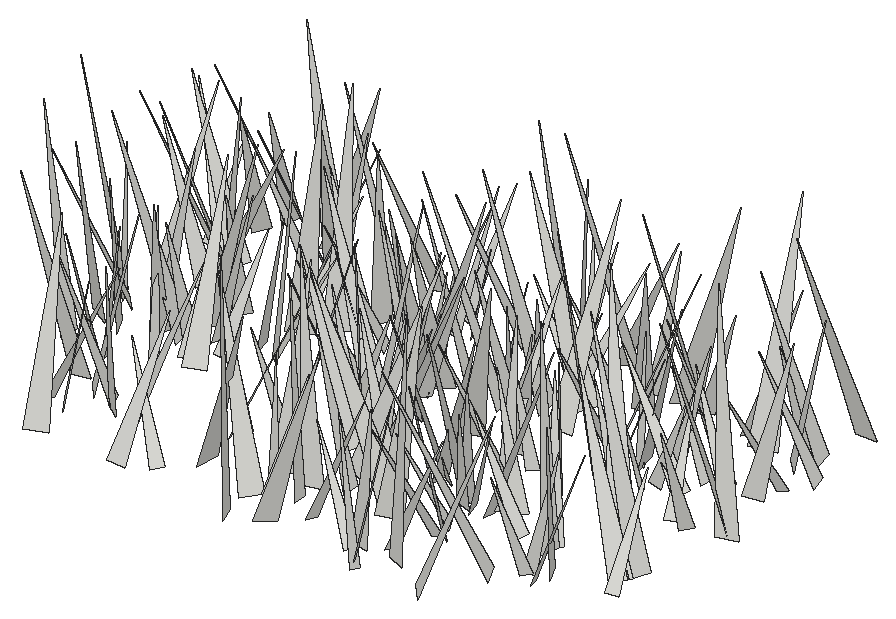
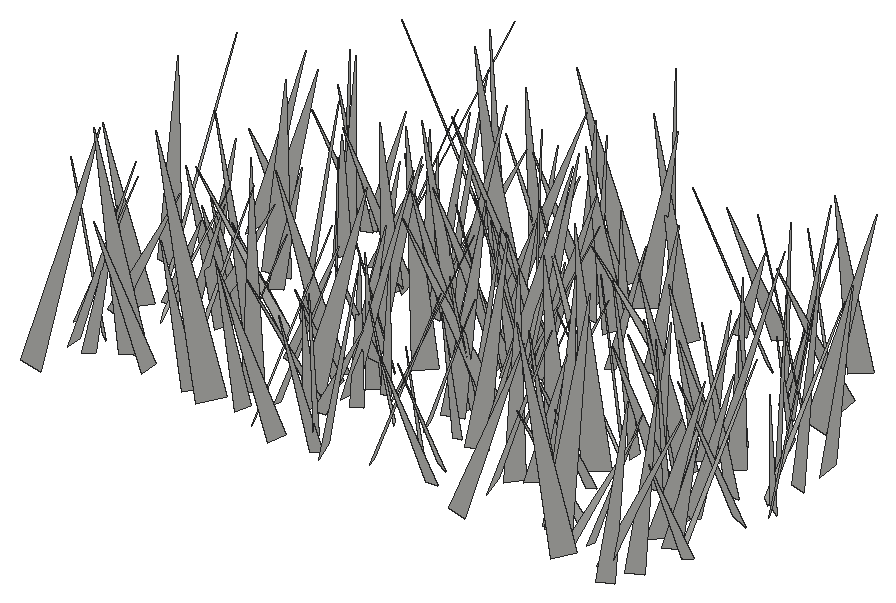
# SketchUp Ruby script. Lengths in inches.
U = 1.inch
M = Sketchup.active_model
def pt(a) = Geom::Point3d.new(a.map { |v| v * U })
def face(e, loops, mat)
  f = e.add_face(loops[0].map { |a| pt(a) })
  loops[1..].each { |l| e.add_face(l.map { |a| pt(a) }).erase! }
  f.material = f.back_material = mat if mat
  f
end
# faces: each face lists its corners as indices into pts; further lists are holes
def faces(e, pts, list, mat = nil) = list.each { |f| face(e, (f[0].is_a?(Array) ? f : [f]).map { |l| l.map { |i| pts[i] } }, mat) }
# xy, xz, yz: faces in a plane at the given z, y or x. An outline is a flat list of corners, or four numbers for a rectangle; further outlines are holes
def ring(l) = l.size == 4 ? [[l[0], l[1]], [l[2], l[1]], [l[2], l[3]], [l[0], l[3]]] : l.each_slice(2).to_a
def flat(e, list, mat, &to3) = list.each { |f| face(e, (f[0].is_a?(Array) ? f : [f]).map { |l| ring(l).map { |u, v| to3.(u, v) } }, mat) }
def xy(e, z, list, mat = nil) = flat(e, list, mat) { |x, y| [x, y, z] }
def xz(e, y, list, mat = nil) = flat(e, list, mat) { |x, z| [x, y, z] }
def yz(e, x, list, mat = nil) = flat(e, list, mat) { |y, z| [x, y, z] }
def lines(e, pts, list) = list.each { |a, b| e.add_line(pt(pts[a]), pt(pts[b])) }
# prism: a flat outline (further loops are holes) pulled along v
def prism(e, loops, v, mat = nil)
  f = face(e, loops, mat); d = Geom::Vector3d.new(v.map { |x| x * U })
  f.pushpull(f.normal.samedirection?(d) ? d.length : -d.length)
end
def box(e, o, s, mat = nil) = prism(e, [[o, [o[0] + s[0], o[1], o[2]], [o[0] + s[0], o[1] + s[1], o[2]], [o[0], o[1] + s[1], o[2]]]], [0, 0, s[2]], mat)
def at(x, y, z, deg = 0) = Geom::Transformation.translation(pt([x, y, z])) * Geom::Transformation.rotation(ORIGIN, Z_AXIS, deg.degrees)
def axes(o, x, y, z) = Geom::Transformation.new([*x, 0, *y, 0, *z, 0, *pt(o).to_a, 1])
def part(name) = M.definitions.add(name)
# library, detail: a bought-in or finely detailed component or shape, given as its bounding box
def library(name, o, s) = part(name).tap { |d| box(d.entities, o, s) }
def detail(e, o, s) = box(e.add_group.entities, o, s)
def put(e, d, t, mat = nil) = e.add_instance(d, t).tap { |i| i.material = mat if mat }
def group(e, t, mat = nil) = e.add_group.tap { |g| g.transformation = t; g.material = mat if mat }.entities
root = M.entities
c1 = part("fur_instance\#9")
p = [[0.8125,0,1.79],[0.67,-0.02,1.48],[0,-0.11,0],[0,0.11,0]]
faces(c1.entities,p,[[0,1,2,3]])
put(root,c1,axes([477.54,253.75,-21.66],[5.60342,-3.67276,1.04707],[-3.81273,-5.48708,1.15708],[-0.22057,1.54484,6.59914]))
put(root,c1,axes([489.59,252.63,-21.66],[4.90909,4.36789,0.50992],[4.39704,-4.86378,-0.66882],[0.06695,-0.83837,6.53684]))
put(root,c1,axes([475.34,252.89,-21.66],[-6.98093,-2.98191,2.95578],[-3.56155,7.24267,-1.10492],[2.22346,2.23913,7.51028]))
put(root,c1,axes([485.04,252.59,-21.66],[-4.58169,-0.00231,0.33908],[-0.10273,4.38765,-1.35823],[0.32316,1.36211,4.37574]))
put(root,c1,axes([483.6,254.77,-21.66],[0.23103,-4.99246,1.62863],[-5.17408,0.0623,0.92493],[0.89778,1.64376,4.91147]))
put(root,c1,axes([483.45,254.25,-21.66],[-2.38468,3.13652,0.12042],[3.02513,2.25628,1.13874],[-0.83714,-0.7813,3.77197]))
put(root,c1,axes([491.6,256.91,-21.66],[-6.74137,-3.47517,0.05647],[-3.44773,6.70195,0.85032],[0.43951,-0.73012,7.53656]))
put(root,c1,axes([484.39,253.45,-21.66],[3.67967,2.76321,1.03507],[2.46473,-3.78797,1.35021],[-1.62229,0.51247,4.39911]))
put(root,c1,axes([466.65,253.6,-21.66],[-1.32926,4.80497,0.97182],[4.66035,1.55098,-1.29408],[1.52094,-0.553,4.81456]))
put(root,c1,axes([460.62,253.74,-21.66],[-3.43213,5.64571,1.59286],[5.69776,3.64732,-0.65059],[1.39526,-1.00684,6.57497]))
put(root,c1,axes([468.8125,254.67,-21.66],[-2.26305,3.25436,0.20739],[3.19812,2.16563,0.91504],[-0.63708,-0.68879,3.8568]))
put(root,c1,axes([486.45,254.625,-21.66],[3.17531,6.56755,2.54139],[6.79761,-3.58673,0.77578],[-1.83954,-1.91744,7.25351]))
put(root,c1,axes([470.55,257.12,-21.66],[6.6655,-1.52718,0.22941],[-1.49066,-6.62814,-0.81212],[-0.40351,-0.74118,6.78982]))
put(root,c1,axes([485.29,255.67,-21.66],[4.11337,-1.35782,0.42666],[-1.42017,-4.00175,0.95638],[-0.09392,1.04301,4.22479]))
put(root,c1,axes([475.1,255.56,-21.66],[-5.2406,4.407,1.34408],[4.57378,5.22157,0.71269],[0.55566,-1.41624,6.81011]))
put(root,c1,axes([479.43,255.63,-21.66],[4.44559,-0.41699,0.42413],[-0.48383,-4.39553,0.74982],[-0.34594,0.78895,4.4017]))
put(root,c1,axes([459.94,257.18,-21.66],[4.41125,2.39111,1.26664],[2.67652,-4.21168,-1.37073],[-0.39751,-1.82353,4.82677]))
put(root,c1,axes([475.95,255.86,-21.66],[1.17442,4.10835,0.87727],[4.16659,-1.02282,-0.78793],[0.5364,-1.0501,4.19964]))
put(root,c1,axes([493.22,258.1875,-21.66],[1.75124,-3.26229,0.83742],[-3.12175,-1.92651,-0.97669],[-1.26432,0.23809,3.57148]))
put(root,c1,axes([486.37,258.55,-21.66],[-0.29394,-4.28793,0.2812],[-4.0742,0.18848,-1.38464],[-1.36614,0.36048,4.06885]))
put(root,c1,axes([486.57,258.94,-21.66],[-3.34858,-4.98605,1.16696],[-4.83329,3.53804,1.24784],[1.69169,0.23891,5.87509]))
put(root,c1,axes([462.59,258.34,-21.66],[-2.53313,-4.37285,1.78451],[-4.47538,2.86942,0.67851],[1.50904,1.16947,5.00781]))
put(root,c1,axes([475.53,256.97,-21.66],[-3.90689,0.46662,1.17538],[0.26281,4.03296,-0.72751],[1.23701,0.61693,3.86682]))
put(root,c1,axes([465.07,256.54,-21.66],[3.93505,4.96293,0.50565],[4.97977,-3.8695,-0.7745],[0.29702,-0.87596,6.28613]))
put(root,c1,axes([462.05,259.17,-21.66],[-5.06877,-1.96642,0.89661],[-1.81084,5.11214,0.97466],[1.17965,-0.60192,5.34876]))
put(root,c1,axes([477.48,256.97,-21.66],[-6.31895,-1.30533,1.91515],[-1.71826,6.37081,-1.32708],[1.5554,1.73484,6.31441]))
put(root,c1,axes([460.6,260.3,-21.66],[-3.28751,-5.48957,1.02333],[-5.33666,3.43821,1.29963],[1.64396,0.18343,6.2653]))
put(root,c1,axes([494.35,259.13,-21.66],[-4.3896,-2.50757,2.34029],[-2.3133,4.97071,0.98703],[2.5325,0.19407,4.95805]))
put(root,c1,axes([458.72,257.25,-21.66],[4.92318,-0.35306,0.35659],[-0.43613,-4.74982,1.31852],[-0.24819,1.34315,4.75646]))
put(root,c1,axes([493.17,258.53,-21.66],[0.04539,-4.24616,1.86431],[-4.44886,0.48634,1.21602],[1.30888,1.80033,4.06857]))
put(root,c1,axes([482.85,258.52,-21.66],[-2.73382,6.12597,3.74599],[6.6709,3.64992,-1.10045],[2.6569,-2.86083,6.61742]))
put(root,c1,axes([486.19,259.98,-21.66],[-3.41179,-1.77285,0.16017],[-1.67154,3.30984,1.02951],[0.61205,-0.84317,3.70451]))
put(root,c1,axes([479.12,259.64,-21.66],[-5.12264,0.34016,1.65759],[0.60899,5.30124,0.79415],[1.57874,-0.94118,5.07212]))
put(root,c1,axes([494.16,257.65,-21.66],[3.89284,1.77366,0.49192],[1.64576,-3.86945,0.92782],[-0.82421,0.65077,4.17603]))
put(root,c1,axes([458.6,260.4,-21.66],[-0.74223,-7.02206,1.66779],[-7.14663,0.48084,-1.156],[-1.00829,1.76103,6.96591]))
put(root,c1,axes([477.17,258.53,-21.66],[-0.74799,6.94474,2.29097],[7.27165,0.46217,0.97314],[-0.77532,-2.36525,6.91678]))
put(root,c1,axes([481.41,260.32,-21.66],[-7.37091,1.53228,0.84327],[1.65266,7.29739,1.18581],[0.57246,-1.33774,7.43452]))
put(root,c1,axes([460.25,259.54,-21.66],[4.87544,3.99495,1.42226],[4.19795,-4.85335,-0.75795],[-0.59966,-1.4959,6.2574]))
put(root,c1,axes([474.77,258.71,-21.66],[-5.03968,3.97301,2.20808],[3.85689,5.48236,-1.06156],[2.40517,-0.46656,6.329]))
put(root,c1,axes([485.34,262.1875,-21.66],[-0.07367,-4.26522,0.50041],[-4.16979,0.19077,1.01214],[1.02732,0.46845,4.14405]))
put(root,c1,axes([469.96,261.27,-21.66],[-0.83956,4.61048,2.28414],[5.1209,0.52371,0.82514],[-0.50027,-2.37653,4.61309]))
put(root,c1,axes([498.55,259.42,-21.66],[-1.96871,3.37657,0.07437],[3.27614,1.93014,-0.90775],[0.82077,0.39482,3.80171]))
put(root,c1,axes([490.25,261.45,-21.66],[-3.73947,1.85603,0.44676],[1.90802,3.6015,1.00834],[-0.06253,-1.10111,4.05114]))
put(root,c1,axes([485.99,262.29,-21.66],[4.14097,0.37336,0.37849],[0.46882,-3.96604,-1.21698],[-0.25072,-1.24957,3.97567]))
put(root,c1,axes([472.2,262.34,-21.66],[-3.76395,0.54517,1.33918],[0.93594,3.7652,1.09781],[1.1021,-1.33566,3.64133]))
put(root,c1,axes([485.17,262.84,-21.66],[0.2797,-5.08952,0.70223],[-5.01624,-0.11848,1.13926],[1.11073,0.74654,4.96825]))
put(root,c1,axes([497.95,260.98,-21.66],[-4.76226,4.46867,0.77555],[4.53262,4.64929,1.04363],[-0.16086,-1.29026,6.44663]))
put(root,c1,axes([492.59,261.12,-21.66],[-6.8831,0.44539,2.18741],[0.27023,7.20464,-0.61666],[2.21588,0.50489,6.86987]))
put(root,c1,axes([482.55,264.125,-21.66],[-2.90954,-6.16313,0.64564],[-6.10361,2.97343,0.8781],[1.07095,0.20243,6.75859]))
put(root,c1,axes([469.79,260.22,-21.66],[4.40688,2.08061,0.00975],[2.02682,-4.29803,1.08102],[-0.47012,0.97349,4.75194]))
put(root,c1,axes([488.1,264.1,-21.66],[-5.70608,-2.81682,0.48614],[-2.67601,5.6456,1.30244],[1.0049,-0.96065,6.22877]))
put(root,c1,axes([483.9,264.02,-21.66],[-1.823,-5.96341,0.88128],[-5.94354,1.93183,0.77754],[1.00658,0.60664,6.18716]))
put(root,c1,axes([482.34,263.86,-21.66],[6.03259,-1.06555,0.38284],[-1.02373,-6.01977,-0.62323],[-0.48366,-0.54868,6.09418]))
put(root,c1,axes([492.49,261.68,-21.66],[-4.5808,2.50643,0.71678],[2.42315,4.62824,-0.69815],[0.96142,0.27723,5.1748]))
put(root,c1,axes([478.18,261.3,-21.66],[3.15625,6.97995,0.87784],[7.00121,-3.02246,-1.14023],[0.68808,-1.26383,7.57506]))
put(root,c1,axes([498.39,262.12,-21.66],[-7.87651,1.28049,0.44694],[1.23259,7.85729,-0.78901],[0.56579,0.70864,7.94081]))
put(root,c1,axes([476.51,263.96,-21.66],[-4.90081,-4.60842,2.76686],[-4.75517,5.4628,0.67611],[2.50627,1.35324,6.69315]))
put(root,c1,axes([488.52,263.48,-21.66],[-2.55012,3.64542,1.48438],[3.93085,2.44958,0.73729],[0.20222,-1.64502,4.38733]))
put(root,c1,axes([487.19,262.31,-21.66],[5.64038,0.84844,0.8162],[0.68974,-5.61874,1.07421],[-0.95409,0.95384,5.60177]))
put(root,c1,axes([478.86,263.42,-21.66],[-2.03282,4.17049,1.29504],[4.34211,1.77825,1.08919],[-0.46493,-1.62705,4.50988]))
put(root,c1,axes([476.25,263.72,-21.66],[-6.01632,2.22797,0.81671],[2.32649,5.97644,0.83455],[0.46722,-1.07014,6.36109]))
put(root,c1,axes([458.35,262.9,-21.66],[-3.5127,-1.06556,1.8883],[-1.54789,3.74984,-0.76344],[1.51826,1.35772,3.59049]))
put(root,c1,axes([487.5,263.29,-21.66],[4.97353,-2.18793,2.98402],[-2.79783,-5.49524,0.634],[-2.42149,1.85546,5.39639]))
put(root,c1,axes([454.93,263.9375,-21.66],[-7.05246,-0.20222,1.59365],[-0.38202,7.18084,-0.77939],[1.56034,0.84409,7.01218]))
put(root,c1,axes([454.98,266.61,-21.66],[-2.48382,-6.27006,1.58629],[-6.2632,2.75568,1.08533],[1.61318,1.04494,6.65621]))
put(root,c1,axes([476.97,265.03,-21.66],[3.46953,-2.67132,1.40146],[-2.94376,-3.4648,0.68347],[-0.65905,1.41311,4.3251]))
put(root,c1,axes([474.43,265.07,-21.66],[3.70527,-2.55389,0.75103],[-2.66189,-3.54115,1.0909],[0.02774,1.32414,4.36593]))
put(root,c1,axes([456.74,266.31,-21.66],[4.97052,1.68586,2.30908],[2.28367,-5.12743,-1.17229],[-1.72012,-1.9358,5.11604]))
put(root,c1,axes([460.83,264.32,-21.66],[0.97276,4.45119,0.9772],[4.35496,-1.20232,1.14148],[-1.3425,-0.67498,4.41093]))
put(root,c1,axes([459.04,267.11,-21.66],[4.90376,-2.85552,0.72078],[-2.73926,-4.93651,-0.92072],[-1.08166,-0.44414,5.59939]))
put(root,c1,axes([475.1,267.5,-21.66],[-5.50457,-1.9976,0.13924],[-1.94432,5.42927,1.02602],[0.47897,-0.91798,5.76524]))
put(root,c1,axes([474.72,265.8,-21.66],[0.57769,-3.84784,2.16026],[-4.16363,-1.197,-1.01866],[-1.46176,1.88882,3.75525]))
put(root,c1,axes([461.22,267.4375,-21.66],[3.60801,-2.69307,1.35493],[-2.4926,-3.85347,-1.02171],[-1.69571,-0.06573,4.3848]))
put(root,c1,axes([470.25,266.47,-21.66],[6.04949,2.12455,0.78775],[2.22415,-5.99674,-0.90711],[-0.43293,-1.1207,6.34722]))
put(root,c1,axes([455.41,268.98,-21.66],[-4.43936,-4.76816,0.23664],[-4.66276,4.39992,1.18262],[1.02469,-0.63608,6.40661]))
put(root,c1,axes([488.52,267.26,-21.66],[3.47548,2.68418,2.07766],[3.24177,-3.50628,-0.89294],[-1.00618,-2.02524,4.29959]))
put(root,c1,axes([460.34,267.6,-21.66],[-7.46338,-1.41905,1.28497],[-1.31215,7.55774,0.72509],[1.39396,-0.48353,7.56241]))
put(root,c1,axes([475.88,266.6,-21.66],[-6.89397,4.20656,1.53795],[4.42912,6.82252,1.19307],[0.66584,-1.82904,7.9874]))
put(root,c1,axes([477.26,265.78,-21.66],[6.02676,-0.13267,0.65935],[-0.25057,-5.95995,1.09109],[-0.62414,1.1116,5.92866]))
put(root,c1,axes([474.29,268.35,-21.66],[-3.67064,-4.64361,1.03864],[-4.58105,3.8034,0.81465],[1.28682,0.29416,5.86285]))
put(root,c1,axes([497.07,268.18,-21.66],[2.57242,-3.23839,0.522],[-3.12857,-2.6216,-0.84629],[-0.98573,-0.13048,4.04824]))
put(root,c1,axes([493.08,267.05,-21.66],[-3.28307,2.60382,1.30489],[2.8552,3.26547,0.66758],[0.57484,-1.34832,4.13676]))
put(root,c1,axes([462.01,265.79,-21.66],[-2.71251,3.20119,0.88639],[3.03008,2.85354,-1.03292],[1.36084,0.02704,4.06674]))
put(root,c1,axes([494.09,265.75,-21.66],[-3.06885,7.2619,1.47031],[7.40414,2.94663,0.90053],[-0.27521,-1.70206,7.83212]))
put(root,c1,axes([480.46,269.07,-21.66],[3.94338,-5.9757,0.15667],[-5.94055,-3.89659,0.90015],[0.66588,0.62564,7.10275]))
put(root,c1,axes([463.16,265.17,-21.66],[-3.56616,5.34471,0.77163],[5.27091,3.64619,-0.89538],[1.17426,-0.13507,6.36253]))
put(root,c1,axes([472.08,268.04,-21.66],[-2.77092,-3.22119,0.17285],[-3.17409,2.68192,-0.90354],[-0.57541,0.71776,4.15182]))
put(root,c1,axes([476.3,265.0625,-21.66],[3.93079,5.90323,1.06815],[5.73682,-4.07234,1.39466],[-1.7544,-0.09002,6.95371]))
put(root,c1,axes([477.33,266,-21.66],[-3.93965,-2.75758,3.63418],[-3.8658,4.56754,-0.72493],[2.42222,2.80458,4.7539]))
put(root,c1,axes([498.85,269.73,-21.66],[-5.87389,-5.06073,1.31002],[-4.91563,6.01764,1.20596],[1.77871,-0.08191,7.65893]))
put(root,c1,axes([485.84,268.02,-21.66],[1.13242,-3.28388,1.61058],[-3.44754,-1.52145,-0.67814],[-1.2216,1.24962,3.40681]))
put(root,c1,axes([484.38,269.12,-21.66],[0.42808,-6.23217,1.75974],[-6.34467,-0.7568,-1.13683],[-1.29687,1.64535,6.14254]))
put(root,c1,axes([463.53,267.12,-21.66],[-0.65991,4.20046,0.70673],[4.09857,0.8209,-1.05196],[1.15975,-0.51096,4.1198]))
put(root,c1,axes([464.65,269.54,-21.66],[5.2345,0.58731,0.96902],[0.7581,-5.21929,-0.93179],[-0.84215,-1.04786,5.18428]))
put(root,c1,axes([476.94,268.65,-21.66],[-3.42512,-4.29344,1.99666],[-4.721,3.28594,-1.03273],[0.36395,2.21827,5.39431]))
put(root,c1,axes([462.21,268.6,-21.66],[4.7492,-0.22527,1.39473],[-0.44396,-4.88167,0.72329],[-1.34124,0.81823,4.6992]))
put(root,c1,axes([489.3,269.375,-21.66],[-5.53788,-5.2946,2.37412],[-5.70348,5.57065,-0.88067],[1.06751,2.29618,7.61087]))
put(root,c1,axes([454.62,269.47,-21.66],[-6.58446,-3.61184,1.85584],[-3.84727,6.67992,-0.64953],[1.29924,1.4758,7.48189]))
put(root,c1,axes([499.61,268.68,-21.66],[-0.81741,7.52572,2.31704],[7.8363,0.54876,0.98214],[-0.77303,-2.39493,7.506]))
put(root,c1,axes([465.74,269.68,-21.66],[3.62695,2.69385,0.06353],[2.59465,-3.4627,-1.30122],[0.7271,-1.08099,4.32648]))
put(root,c1,axes([460.81,269.43,-21.66],[6.40804,-1.16691,1.44574],[-1.35043,-6.49108,0.74636],[-1.27601,1.00946,6.47052]))
put(root,c1,axes([457.27,269.79,-21.66],[1.6675,5.06938,1.93589],[5.41393,-1.41673,-0.95346],[0.36831,-2.12629,5.25072]))
put(root,c1,axes([495.77,268.32,-21.66],[-2.69846,2.82224,0.09608],[2.72603,2.63813,-0.93001],[0.73688,0.57546,3.79233]))
put(root,c1,axes([466.2,268.77,-21.66],[3.82909,4.88275,1.88302],[4.81565,-4.20088,1.10051],[-2.04855,-0.74856,6.10673]))
put(root,c1,axes([475.77,272.38,-21.66],[3.11864,-5.68803,0.55795],[-5.6529,-3.16353,-0.65398],[-0.84244,0.17118,6.45383]))
put(root,c1,axes([454.52,269.46,-21.66],[1.72426,4.07776,1.35625],[4.04188,-2.03524,0.98061],[-1.4597,-0.81871,4.31736]))
put(root,c1,axes([492.26,269.99,-21.66],[-3.43885,-1.25141,0.28396],[-1.28081,3.29756,-0.97876],[-0.07859,1.01608,3.52615]))
put(root,c1,axes([481.72,270.36,-21.66],[3.27603,2.91205,0.73309],[2.99826,-3.11162,-1.03833],[0.1671,-1.26001,4.25844]))
put(root,c1,axes([461.38,271.9,-21.66],[3.51488,-3.51732,0.75482],[-3.443,-3.59499,-0.71937],[-1.04262,0.01399,4.9202]))
put(root,c1,axes([492.47,270.95,-21.66],[0.8957,-3.44027,0.95903],[-3.38159,-0.49886,1.36875],[1.14894,1.21373,3.28089]))
put(root,c1,axes([494.3,271.09,-21.66],[-4.30239,2.31555,0.00735],[2.25428,4.18495,1.12996],[-0.52922,-0.99839,4.75348]))
put(root,c1,axes([475.25,271.13,-21.66],[1.48907,3.83094,1.46531],[4.09712,-1.31638,-0.722],[0.19182,-1.62223,4.04625]))
put(root,c1,axes([475.52,270.61,-21.66],[6.84778,-1.68967,1.39359],[-1.92956,-6.81846,1.21431],[-1.03628,1.53061,6.94784]))
put(root,c1,axes([490.17,269.98,-21.66],[3.37937,2.22818,0.23171],[2.15143,-3.34494,0.78826],[-0.62436,0.53406,3.97033]))
put(root,c1,axes([490.44,272.5625,-21.66],[6.84395,0.46131,0.76105],[0.6015,-6.74756,-1.31919],[-0.65589,-1.3745,6.73144]))
put(root,c1,axes([481.35,272.72,-21.66],[1.83451,-3.56347,0.05806],[-3.52397,-1.80394,0.62811],[0.53227,0.33851,3.95843]))
put(root,c1,axes([480.33,272.86,-21.66],[-0.97115,-4.17934,0.95629],[-4.09852,1.19278,1.05068],[1.25838,0.65947,4.16006]))
put(root,c1,axes([474.66,269.95,-21.66],[6.67299,1.88656,0.54903],[1.75109,-6.59185,1.3677],[-0.89119,1.17381,6.79833]))
put(root,c1,axes([487.18,273.16,-21.66],[-0.13278,-3.81265,0.23397],[-3.74221,0.08288,-0.77308],[-0.76609,0.25594,3.73581]))
put(root,c1,axes([465.32,272.23,-21.66],[-3.47226,6.33449,3.63746],[6.89094,4.17667,-0.69553],[2.42317,-2.80055,7.19017]))
put(root,c1,axes([492.625,272.375,-21.66],[4.10289,-2.86128,0.97197],[-3.01034,-4.01302,0.89377],[-0.2636,1.29386,4.92156]))
put(root,c1,axes([472.33,274.5,-21.66],[3.11347,-5.57932,0.56956],[-5.54553,-3.1599,-0.63956],[-0.83685,0.18197,6.35716]))
put(root,c1,axes([470.2,274.02,-21.66],[-4.41173,-1.92667,0.46008],[-1.77307,4.34177,1.17998],[0.88316,-0.90777,4.66723]))
put(root,c1,axes([494.55,273.2,-21.66],[-3.60372,1.36671,1.25031],[1.68423,3.55609,0.96723],[0.77106,-1.37995,3.73084]))
put(root,c1,axes([458.37,274.59,-21.66],[-4.85913,-4.7221,0.69622],[-4.68141,4.90862,0.61965],[0.93132,0.03646,6.74725]))
put(root,c1,axes([496.72,272.31,-21.66],[-1.92431,3.57441,0.40694],[3.46774,1.72017,1.28872],[-0.95749,-0.95373,3.84949]))
put(root,c1,axes([479.86,272.625,-21.66],[-7.1325,-1.97369,0.04131],[-1.9512,7.0246,-1.27181],[-0.29997,1.23662,7.29044]))
put(root,c1,axes([457.51,273.25,-21.66],[-4.78062,2.36193,1.12593],[2.54726,4.73726,0.87783],[0.59826,-1.2963,5.25951]))
put(root,c1,axes([490.34,272.22,-21.66],[1.055,3.81063,1.04337],[3.83467,-1.24762,0.6792],[-0.95124,-0.80317,3.89521]))
put(root,c1,axes([489.08,270.9,-21.66],[5.73522,3.47371,0.17785],[3.39582,-5.66618,1.16354],[-0.75282,0.90483,6.60345]))
put(root,c1,axes([481.44,271.6,-21.66],[-0.33332,4.6985,0.41104],[4.65173,0.39553,-0.74898],[0.77866,-0.35159,4.65038]))
put(root,c1,axes([496.18,273.67,-21.66],[-4.80301,-2.64529,0.12183],[-2.62964,4.73476,-0.865],[-0.31202,0.81591,5.41463]))
put(root,c1,axes([481.99,274.17,-21.66],[-7.83608,-0.63477,1.59162],[-0.4911,7.96997,0.76075],[1.64165,-0.64574,7.82485]))
put(root,c1,axes([497.83,273.28,-21.66],[-1.7832,4.7887,2.83203],[5.02838,2.65983,-1.33139],[2.38064,-2.03113,4.93345]))
put(root,c1,axes([472.91,272.79,-21.66],[-4.76571,-0.2474,0.30777],[-0.30187,4.68534,-0.90794],[0.25457,0.92426,4.68496]))
put(root,c1,axes([498.58,275.11,-21.66],[-0.19761,-4.29399,0.26182],[-4.09062,0.10641,-1.34218],[-1.33181,0.31028,4.08362]))
put(root,c1,axes([480.77,274.98,-21.66],[0.8236,-4.35079,0.44599],[-4.32851,-0.74586,0.71716],[0.62636,0.56649,4.3696]))
put(root,c1,axes([473.95,274.25,-21.66],[-0.58036,-3.55618,1.37675],[-3.59236,0.97706,1.00942],[1.27936,1.13031,3.45894]))
put(root,c1,axes([457.67,274.07,-21.66],[5.28703,-2.12696,0.17156],[-2.11759,-5.17319,1.12251],[0.26309,1.10465,5.58719]))
put(root,c1,axes([455.2,271.72,-21.66],[2.05142,5.93925,0.09208],[5.90467,-2.04959,0.65232],[-0.64654,0.12643,6.2496]))
put(root,c1,axes([484.12,272.59,-21.66],[-1.25446,7.26591,1.58891],[7.27727,1.53186,-1.25954],[1.53602,-1.32352,7.26503]))
put(root,c1,axes([476.24,274.125,-21.66],[-5.31837,-1.43549,0.4315],[-1.49067,5.23198,-0.96754],[0.15722,1.04767,5.42306]))
put(root,c1,axes([483.2,273.55,-21.66],[3.56009,0.21869,0.65734],[0.01468,-3.46445,1.07311],[-0.69261,1.05069,3.40155]))
put(root,c1,axes([455.43,276.81,-21.66],[-4.61159,-4.4726,0.38091],[-4.39573,4.61032,0.9157],[0.90928,-0.396,6.35865]))
put(root,c1,axes([466.86,273.61,-21.66],[-5.99811,4.4385,2.51735],[4.45899,6.44808,-0.74453],[2.48087,-0.8583,7.4245]))
put(root,c1,axes([468.24,276.1,-21.66],[5.51508,-3.1001,1.56666],[-3.03836,-5.73026,-0.64316],[-1.68328,0.18611,6.29389]))
put(root,c1,axes([477.88,275.12,-21.66],[3.15545,2.01724,0.79775],[2.15051,-3.09372,-0.68323],[-0.2846,-1.01105,3.6823]))
put(root,c1,axes([464.3,273.96,-21.66],[0.4921,4.23207,0.57816],[4.10963,-0.31046,-1.22532],[1.16432,-0.69285,4.08059]))
put(root,c1,axes([483.78,275.44,-21.66],[-6.02527,4.37662,1.94606],[4.73834,5.90349,1.39383],[0.70004,-2.28907,7.31546]))
put(root,c1,axes([486.54,277.32,-21.66],[1.84605,-6.6162,0.27609],[-6.51912,-1.76548,1.28157],[1.16252,0.60597,6.74831]))
put(root,c1,axes([456.93,275.94,-21.66],[3.49606,4.56093,2.47636],[5.16488,-3.35013,-1.12142],[-0.50841,-2.67048,5.63622]))
put(root,c1,axes([467.35,275.55,-21.66],[-4.02277,2.62654,1.01722],[2.78428,3.97624,0.74391],[0.42575,-1.18612,4.74637]))
put(root,c1,axes([499.65,277.03,-21.66],[-4.7933,-0.97536,0.74224],[-0.77682,4.73507,1.20565],[0.94805,-1.05153,4.74061]))
put(root,c1,axes([484.64,277.49,-21.66],[-4.25051,-1.02119,0.70994],[-0.79222,4.17184,1.25768],[0.95876,-1.08007,4.18663]))
put(root,c1,axes([462.7,278.96,-21.66],[5.93446,-4.51627,0.11992],[-4.41947,-5.84426,-1.3935],[-0.93776,-1.03771,7.32616]))
put(root,c1,axes([457.64,276.26,-21.66],[-5.5849,2.54638,0.93821],[2.66389,5.55377,0.78405],[0.51763,-1.10771,6.08773]))
put(root,c1,axes([482.02,276.86,-21.66],[-2.52559,2.65872,0.46687],[2.62617,2.27215,1.26725],[-0.62447,-1.19747,3.44114]))
put(root,c1,axes([491.17,277.58,-21.66],[-5.74367,-4.09689,1.01684],[-4.21686,5.6466,-1.0688],[0.19121,1.46278,6.97366]))
put(root,c1,axes([464.03,277.34,-21.66],[-1.49797,-4.88201,2.75569],[-5.27998,2.18724,1.00478],[1.88406,2.24805,5.00683]))
put(root,c1,axes([497.22,277.68,-21.66],[4.01593,3.70117,1.52807],[3.99587,-3.8439,-1.19115],[-0.25835,-1.92018,5.32987]))
put(root,c1,axes([482.36,276.15,-21.66],[1.65691,4.63189,0.02775],[4.518,-1.60961,-1.09423],[1.0212,-0.39403,4.79608]))
put(root,c1,axes([476.14,279.38,-21.66],[-5.06216,-2.56794,0.53616],[-2.44101,5.03776,1.08155],[0.96086,-0.73072,5.57226]))
put(root,c1,axes([473.18,278.28,-21.66],[3.34183,1.38887,0.77255],[1.56239,-3.2005,-1.00466],[-0.29109,-1.23347,3.4767]))
put(root,c1,axes([456.21,276.67,-21.66],[-3.43494,4.07646,0.13435],[4.04677,3.38429,0.77755],[-0.50915,-0.60283,5.27368]))
put(root,c1,axes([460.22,279.14,-21.66],[-4.26767,-0.91045,0.71231],[-0.70932,4.21373,1.13607],[0.91278,-0.98229,4.21323]))
put(root,c1,axes([468.82,277.41,-21.66],[-7.05105,-1.29004,0.36767],[-1.33665,6.92247,-1.34515],[0.11284,1.38992,7.04075]))
put(root,c1,axes([496.81,279.64,-21.66],[3.89618,-1.88557,1.1779],[-1.51971,-3.99347,-1.36592],[-1.62275,-0.78732,4.1073]))
put(root,c1,axes([454.74,277.03,-21.66],[-0.81178,3.59213,0.55552],[3.51446,0.92094,-0.81938],[0.92765,-0.34562,3.5904]))
put(root,c1,axes([498.1875,279.27,-21.66],[-6.30832,-1.1114,1.05664],[-1.00602,6.37534,0.69964],[1.15742,-0.51611,6.36715]))
put(root,c1,axes([456.05,280.31,-21.66],[3.84252,-3.67557,0.42443],[-3.56655,-3.84235,-0.9854],[-0.98471,-0.42605,5.2253]))
put(root,c1,axes([482.69,276.93,-21.66],[-4.63028,1.37895,0.71291],[1.15549,4.55932,-1.31404],[1.03661,1.07721,4.64912]))
put(root,c1,axes([461.4,279.38,-21.66],[-3.04212,-3.44962,0.11938],[-3.35963,2.92271,-1.15727],[-0.79185,0.85236,4.45141]))
put(root,c1,axes([489.52,279.42,-21.66],[3.13596,-3.23192,0.2957],[-3.22644,-3.06024,0.76944],[0.35051,0.74607,4.43707]))
put(root,c1,axes([462.7,279.11,-21.66],[1.59006,-7.38899,3.46765],[-7.94346,-2.21328,-1.07372],[-1.87702,3.10714,7.48148]))
put(root,c1,axes([487.81,279.6,-21.66],[6.25642,-5.32962,1.03257],[-5.42827,-6.12142,1.29455],[0.06986,1.65444,8.11614]))
put(root,c1,axes([462.29,277.35,-21.66],[4.05537,2.07279,0.17475],[1.9711,-3.95155,1.12829],[-0.66463,0.92835,4.41242]))
put(root,c1,axes([472.55,277.45,-21.66],[1.79845,4.31058,0.12569],[4.2592,-1.79684,0.67963],[-0.67534,0.14702,4.621]))
put(root,c1,axes([468.5,281.09,-21.66],[-0.3519,-5.66898,0.64957],[-5.59847,0.21723,-1.13712],[-1.1029,0.70611,5.5649]))
put(root,c1,axes([484.61,279.5,-21.66],[-7.32124,-3.15954,0.71739],[-3.23761,7.2018,-1.32279],[0.12329,1.49974,7.86343]))
put(root,c1,axes([485.79,279.21,-21.66],[4.38322,-1.64948,1.59394],[-1.93146,-4.50849,0.64578],[-1.2373,1.19448,4.63858]))
put(root,c1,axes([494.61,278.2,-21.66],[-2.78975,7.45432,2.27613],[7.61508,3.12201,-0.8911],[1.66081,-1.79348,7.90921]))
put(root,c1,axes([492.91,278.99,-21.66],[5.00649,-0.69371,1.01239],[-0.92226,-4.93206,1.18126],[-0.80969,1.32843,4.91435]))
put(root,c1,axes([456.72,282.15,-21.66],[4.17409,-3.35782,0.27535],[-3.2273,-4.11088,-1.20788],[-0.96712,-0.77425,5.2191]))
put(root,c1,axes([457.68,281.42,-21.66],[-3.27123,-4.88451,0.3113],[-4.82797,3.15879,-1.17003],[-0.80376,0.90546,5.76111]))
put(root,c1,axes([460.55,281.2,-21.66],[5.42547,-4.53511,0.52895],[-4.56014,-5.3411,0.98008],[0.2284,1.09004,7.00303]))
put(root,c1,axes([471.8,279.32,-21.66],[0.88242,4.55252,0.64978],[4.54635,-0.76413,-0.82042],[0.6916,-0.78549,4.5641]))
put(root,c1,axes([480.07,279.56,-21.66],[-4.86729,-1.78674,2.25978],[-2.35287,5.02555,-1.09424],[1.66225,1.88173,5.06809]))
put(root,c1,axes([479.28,280.55,-21.66],[0.33455,3.97904,1.71347],[4.11253,0.24873,-1.38056],[1.36232,-1.72801,3.74683]))
put(root,c1,axes([482.08,280.74,-21.66],[4.93305,-2.19664,0.15391],[-2.18894,-4.85066,0.92924],[0.23965,0.9109,5.31946]))
put(root,c1,axes([478.96,280.29,-21.66],[-6.73527,-1.87686,1.53677],[-2.12146,6.75676,-1.04577],[1.17629,1.43931,6.91323]))
put(root,c1,axes([498.45,282.94,-21.66],[-0.93689,-7.58778,0.99671],[-7.63501,0.85799,-0.64504],[-0.52389,1.06539,7.61814]))
